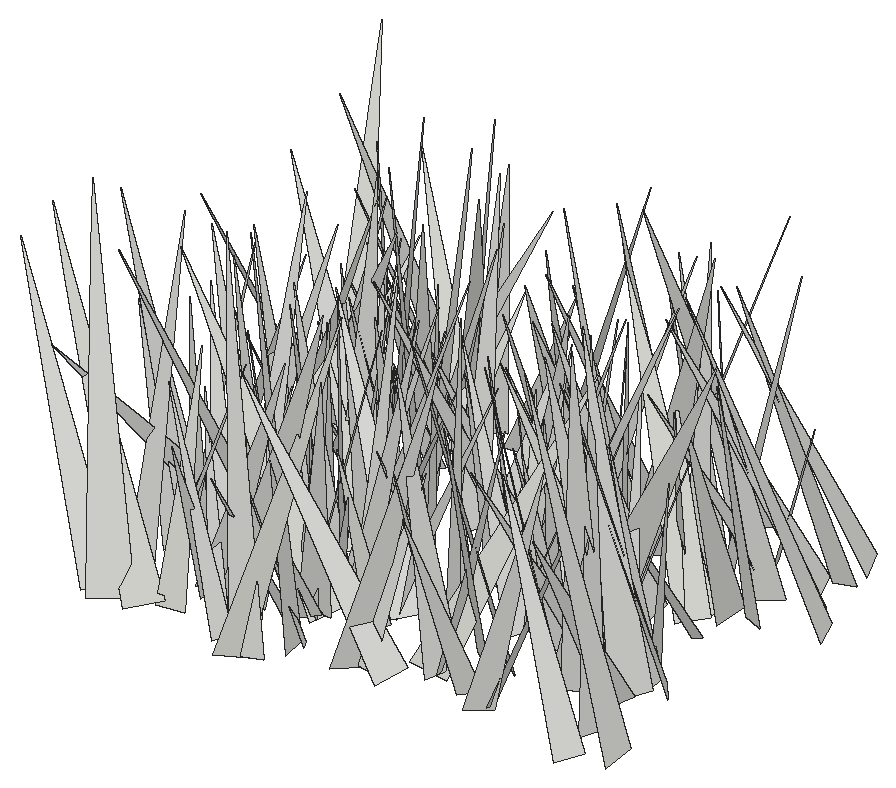
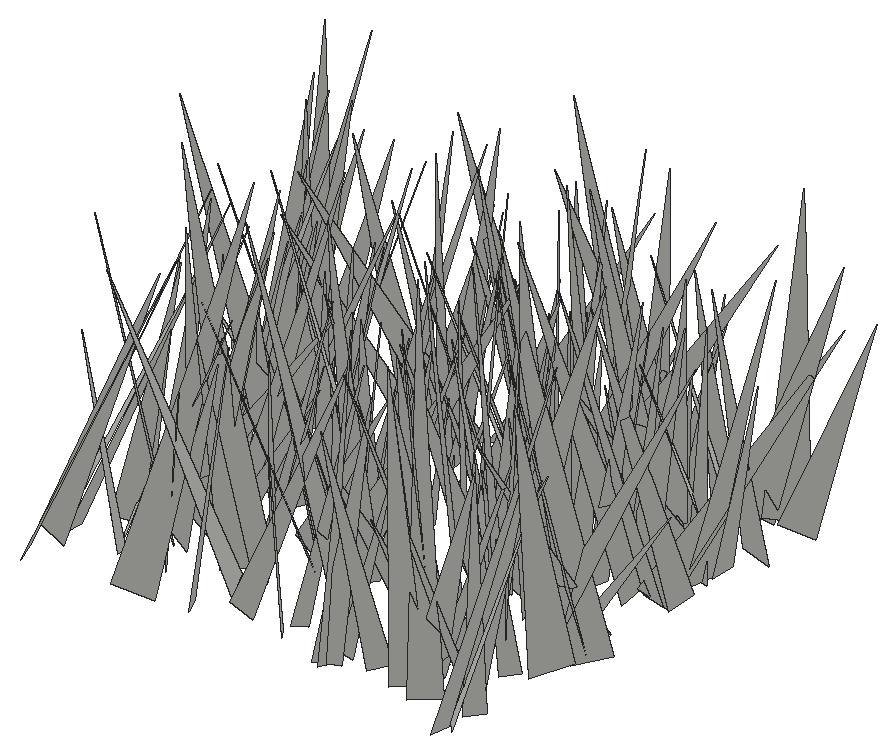
# SketchUp Ruby script. Lengths in inches.
U = 1.inch
M = Sketchup.active_model
def pt(a) = Geom::Point3d.new(a.map { |v| v * U })
def face(e, loops, mat)
  f = e.add_face(loops[0].map { |a| pt(a) })
  loops[1..].each { |l| e.add_face(l.map { |a| pt(a) }).erase! }
  f.material = f.back_material = mat if mat
  f
end
# faces: each face lists its corners as indices into pts; further lists are holes
def faces(e, pts, list, mat = nil) = list.each { |f| face(e, (f[0].is_a?(Array) ? f : [f]).map { |l| l.map { |i| pts[i] } }, mat) }
# xy, xz, yz: faces in a plane at the given z, y or x. An outline is a flat list of corners, or four numbers for a rectangle; further outlines are holes
def ring(l) = l.size == 4 ? [[l[0], l[1]], [l[2], l[1]], [l[2], l[3]], [l[0], l[3]]] : l.each_slice(2).to_a
def flat(e, list, mat, &to3) = list.each { |f| face(e, (f[0].is_a?(Array) ? f : [f]).map { |l| ring(l).map { |u, v| to3.(u, v) } }, mat) }
def xy(e, z, list, mat = nil) = flat(e, list, mat) { |x, y| [x, y, z] }
def xz(e, y, list, mat = nil) = flat(e, list, mat) { |x, z| [x, y, z] }
def yz(e, x, list, mat = nil) = flat(e, list, mat) { |y, z| [x, y, z] }
def lines(e, pts, list) = list.each { |a, b| e.add_line(pt(pts[a]), pt(pts[b])) }
# prism: a flat outline (further loops are holes) pulled along v
def prism(e, loops, v, mat = nil)
  f = face(e, loops, mat); d = Geom::Vector3d.new(v.map { |x| x * U })
  f.pushpull(f.normal.samedirection?(d) ? d.length : -d.length)
end
def box(e, o, s, mat = nil) = prism(e, [[o, [o[0] + s[0], o[1], o[2]], [o[0] + s[0], o[1] + s[1], o[2]], [o[0], o[1] + s[1], o[2]]]], [0, 0, s[2]], mat)
def at(x, y, z, deg = 0) = Geom::Transformation.translation(pt([x, y, z])) * Geom::Transformation.rotation(ORIGIN, Z_AXIS, deg.degrees)
def axes(o, x, y, z) = Geom::Transformation.new([*x, 0, *y, 0, *z, 0, *pt(o).to_a, 1])
def part(name) = M.definitions.add(name)
# library, detail: a bought-in or finely detailed component or shape, given as its bounding box
def library(name, o, s) = part(name).tap { |d| box(d.entities, o, s) }
def detail(e, o, s) = box(e.add_group.entities, o, s)
def put(e, d, t, mat = nil) = e.add_instance(d, t).tap { |i| i.material = mat if mat }
def group(e, t, mat = nil) = e.add_group.tap { |g| g.transformation = t; g.material = mat if mat }.entities
root = M.entities
c1 = part("fur_instance\#9")
p = [[0.8125,0,1.79],[0.67,-0.02,1.48],[0,-0.11,0],[0,0.11,0]]
faces(c1.entities,p,[[0,1,2,3]])
put(root,c1,axes([68.28,290.38,-27.1],[4.10212,-1.60455,0.85508],[-1.23063,-4.00368,-1.60913],[-1.3384,-1.23658,4.10033]))
put(root,c1,axes([70.8,287.91,-27.1],[-4.9286,0.63717,0.02707],[0.62924,4.89286,-0.60144],[0.10377,0.59304,4.93308]))
put(root,c1,axes([65.69,287.62,-27.1],[-4.19179,6.94453,1.88873],[7.18228,4.17546,0.58769],[0.45687,-1.92457,8.09026]))
put(root,c1,axes([80.6,290.35,-27.1],[1.77342,-4.13167,0.71101],[-4.001,-1.89854,-1.053],[-1.2523,0.21471,4.37115]))
put(root,c1,axes([77.55,289.49,-27.1],[-6.03456,2.61232,0.13904],[2.52964,5.73798,1.98392],[-0.66667,-1.87372,6.2693]))
put(root,c1,axes([71.93,286.99,-27.1],[6.32729,-2.1008,2.73388],[-3.01636,-6.1404,2.26257],[-1.67006,3.13117,6.27127]))
put(root,c1,axes([86.57,288.8,-27.1],[-4.85696,2.92878,0.85344],[3.03677,4.79447,0.82904],[0.29007,-1.15391,5.61075]))
put(root,c1,axes([72.45,287.27,-27.1],[0.0482,8.00911,1.76337],[7.92916,-0.49572,2.03478],[-2.09374,-1.69294,7.74648]))
put(root,c1,axes([72.46,290.14,-27.1],[-0.70477,-3.63934,0.22038],[-3.52996,0.62491,-0.96896],[-0.91253,0.39339,3.57807]))
put(root,c1,axes([67.9375,288.38,-27.1],[-1.16882,5.10436,1.64073],[5.31118,1.33199,-0.3603],[0.7334,-1.51127,5.22406]))
put(root,c1,axes([64.84,288.08,-27.1],[-3.24359,5.98487,0.42852],[5.75195,2.96279,2.1587],[-1.708,-1.38792,6.45597]))
put(root,c1,axes([66.96,288.01,-27.1],[-3.17251,7.14398,0.8627],[6.87917,2.73438,2.65436],[-2.11131,-1.82544,7.35225]))
put(root,c1,axes([73.53,289.39,-27.1],[-3.08913,-1.9262,0.20442],[-1.91689,2.98464,-0.84391],[-0.27849,0.82245,3.5413]))
put(root,c1,axes([69.64,290.49,-27.1],[3.88235,-7.18309,1.19208],[-7.15051,-3.50623,2.16032],[1.37403,2.04942,7.87416]))
put(root,c1,axes([75.89,289.04,-27.1],[6.31096,-2.97385,1.65761],[-3.28181,-6.24286,1.29466],[-0.9062,1.89806,6.85536]))
put(root,c1,axes([66.57,289.49,-27.1],[4.70564,3.18962,0.73071],[3.27223,-4.59158,-1.02983],[-0.01227,-1.26267,5.59072]))
put(root,c1,axes([87.99,289.93,-27.1],[-7.83982,-0.95667,1.33619],[-0.96404,7.9519,0.03699],[1.33088,0.12461,7.89789]))
put(root,c1,axes([81.66,289.57,-27.1],[4.65487,-3.05281,1.35089],[-3.29302,-4.57961,0.99778],[-0.54826,1.58741,5.47649]))
put(root,c1,axes([73.37,288.93,-27.1],[-7.60319,-2.30719,2.08818],[-2.71089,7.61771,-1.45385],[1.52798,2.03457,7.8114]))
put(root,c1,axes([76.24,289.36,-27.1],[-0.49271,4.25835,1.65602],[4.30491,0.99075,-1.26683],[1.53091,-1.41548,4.0953]))
put(root,c1,axes([68.3,290.51,-27.1],[3.9818,-4.86666,0.84742],[-4.90357,-3.76221,1.43455],[0.59785,1.55519,6.12218]))
put(root,c1,axes([78.86,290.92,-27.1],[-5.74569,2.33772,2.68731],[2.89131,6.03979,0.92776],[2.08013,-1.9379,6.13328]))
put(root,c1,axes([72.27,291.53,-27.1],[1.6892,-5.96403,1.00433],[-6.01842,-1.55459,0.89085],[0.59746,1.20222,6.13428]))
put(root,c1,axes([85.42,293.22,-27.1],[4.02503,-3.95124,0.17731],[-3.62061,-3.78264,-2.10414],[-1.59215,-1.38705,5.23314]))
put(root,c1,axes([77.93,292.04,-27.1],[-3.99319,-2.60087,1.40659],[-2.16034,4.18012,1.59628],[2.0189,-0.6713,4.49021]))
put(root,c1,axes([69.52,289.24,-27.1],[-0.27528,4.26527,0.41219],[4.05575,0.12601,1.40472],[-1.38323,-0.47937,4.03672]))
put(root,c1,axes([72.34,291.2,-27.1],[-3.051,-7.21191,1.32168],[-6.61753,2.09219,-3.8598],[-3.15701,2.58422,6.81338]))
put(root,c1,axes([79.625,292.39,-27.1],[-2.94569,-5.43055,1.36405],[-5.282,3.20651,1.35919],[1.85796,0.50597,6.02666]))
put(root,c1,axes([74.94,292.03,-27.1],[3.15907,-2.58161,1.45094],[-2.40771,-3.47422,-0.93937],[-1.72421,0.12146,3.97014]))
put(root,c1,axes([71.92,291.46,-27.1],[2.13967,5.72529,2.72362],[6.33838,-1.99885,-0.77766],[-0.14822,-2.82858,6.06237]))
put(root,c1,axes([72.78,291.84,-27.1],[-6.95314,3.37085,0.59923],[3.40426,6.66259,2.02209],[-0.36434,-2.07731,7.45788]))
put(root,c1,axes([72.22,292.96,-27.1],[-0.71595,-3.844,0.50308],[-3.36107,0.87042,1.86752],[1.93201,0.08975,3.4353]))
put(root,c1,axes([68.78,290.76,-27.1],[3.00603,-4.02582,3.59921],[-4.80148,-3.87769,-0.32715],[-2.47129,2.63706,5.01362]))
put(root,c1,axes([78.77,291.2,-27.1],[5.20805,0.62891,1.21236],[0.54515,-5.33937,0.42794],[-1.25226,0.29119,5.2284]))
put(root,c1,axes([65.85,295.35,-27.1],[3.04305,-5.48081,0.27728],[-4.42438,-2.6378,-3.58374],[-3.24669,-1.54241,5.14356]))
put(root,c1,axes([80.59,292.77,-27.1],[-4.6315,-5.30606,1.24554],[-5.44783,4.55599,-0.84886],[0.16366,1.49838,6.99175]))
put(root,c1,axes([83.85,293.1,-27.1],[3.80262,-6.94068,2.14426],[-7.19034,-3.9408,-0.00453],[-1.0344,1.87826,7.9141]))
put(root,c1,axes([70.47,289.55,-27.1],[0.64716,8.27924,1.09317],[8.31403,-0.74193,0.69715],[-0.78591,-1.0312,8.27518]))
put(root,c1,axes([71.38,292.79,-27.1],[2.3019,2.88607,2.09295],[3.52279,-2.224,-0.8077],[-0.54756,-2.17555,3.60219]))
put(root,c1,axes([64.86,290.47,-27.1],[1.29784,6.7007,1.25957],[6.74597,-1.44798,0.75208],[-0.98888,-1.08363,6.78367]))
put(root,c1,axes([81.89,295.59,-27.1],[-4.9139,-3.74374,0.55427],[-3.15126,4.55055,2.79845],[2.0958,-1.9355,5.50733]))
put(root,c1,axes([78.78,291.56,-27.1],[2.86323,5.98862,2.41998],[6.20716,-3.28322,0.78076],[-1.78634,-1.80966,6.59182]))
put(root,c1,axes([86.06,290.8125,-27.1],[-7.47088,0.3057,1.86762],[-0.12287,7.51123,-1.721],[1.88848,1.69808,7.27638]))
put(root,c1,axes([82.6,293.33,-27.1],[0.98375,-3.96673,0.69714],[-3.91068,-0.76919,1.14174],[0.96305,0.9285,3.92417]))
put(root,c1,axes([77.86,292.07,-27.1],[-5.58164,-0.15602,0.84627],[-0.25003,5.60842,-0.61509],[0.82341,0.64537,5.54984]))
put(root,c1,axes([70.68,294.19,-27.1],[-2.8459,-6.01928,1.64103],[-5.98512,3.14324,1.14988],[1.76154,0.95508,6.5581]))
put(root,c1,axes([73.4,292.625,-27.1],[2.35807,6.09522,2.44102],[6.53945,-1.94795,-1.45322],[0.58808,-2.77931,6.37184]))
put(root,c1,axes([81.83,290.06,-27.1],[5.28462,2.45266,0.54887],[2.09175,-5.00051,2.20534],[-1.39334,1.79538,5.39252]))
put(root,c1,axes([65.07,292.19,-27.1],[-4.79431,0.50788,0.77321],[0.45097,4.84644,-0.38709],[0.80772,0.30866,4.80557]))
put(root,c1,axes([82.95,292.87,-27.1],[-4.95008,-4.07189,1.35786],[-4.2827,4.82407,-1.14641],[0.2873,1.75371,6.30629]))
put(root,c1,axes([65.53,293.16,-27.1],[1.09401,4.63876,2.44173],[5.21296,-1.22556,-0.00737],[-0.55243,-2.37843,4.76601]))
put(root,c1,axes([78.37,290.66,-27.1],[-2.47927,6.31853,1.78834],[5.49074,3.04318,-3.14001],[3.60191,-0.28983,6.01756]))
put(root,c1,axes([65.26,293.36,-27.1],[-7.08698,0.49693,1.41438],[0.58095,7.2106,0.37757],[1.38199,-0.48283,7.09434]))
put(root,c1,axes([84.66,293.85,-27.1],[-2.85824,2.70123,1.97363],[3.21945,2.92659,0.65696],[0.90938,-1.87078,3.87745]))
put(root,c1,axes([68.97,293.72,-27.1],[3.31439,2.62679,2.62231],[3.03004,-3.94532,0.12232],[-2.14367,-1.5153,4.22732]))
put(root,c1,axes([75.84,294.84,-27.1],[-3.61169,-1.5954,0.61372],[-1.41522,3.59542,1.01805],[0.9587,-0.70282,3.81487]))
put(root,c1,axes([85.44,293.875,-27.1],[-6.5147,3.53544,2.59254],[3.94464,6.75335,0.70282],[1.91322,-1.88542,7.3788]))
put(root,c1,axes([71.05,294.2,-27.1],[1.22573,-5.85041,2.29876],[-6.17569,-1.55733,-0.67049],[-1.1715,2.08841,5.93971]))
put(root,c1,axes([83.51,294.98,-27.1],[3.66547,-5.8791,2.24711],[-5.89364,-4.11869,-1.16204],[-2.20868,1.23351,6.83002]))
put(root,c1,axes([71,294.77,-27.1],[5.57047,2.74276,2.66238],[3.42235,-5.67452,-1.31471],[-1.7025,-2.43273,6.06831]))
put(root,c1,axes([74.32,293.71,-27.1],[4.41432,4.17138,0.78555],[4.1779,-4.06951,-1.86761],[0.75011,-1.88212,5.77916]))
put(root,c1,axes([67.03,291.81,-27.1],[-1.28039,5.01222,0.36244],[4.5705,1.31696,-2.06622],[2.08908,0.19072,4.74262]))
put(root,c1,axes([84.68,296.38,-27.1],[-3.9391,-6.11846,0.96009],[-6.01065,4.05101,1.1555],[1.49311,0.1661,7.18449]))
put(root,c1,axes([81.25,295,-27.1],[0.8668,-4.44855,1.11397],[-4.54098,-0.99091,-0.42373],[-0.6404,1.00517,4.51236]))
put(root,c1,axes([86.24,295.04,-27.1],[-5.08924,-4.37631,0.84531],[-4.44671,5.07308,-0.50754],[0.30556,0.93743,6.69289]))
put(root,c1,axes([66.2,291.19,-27.1],[3.80784,5.11048,0.67094],[4.57882,-3.73693,2.47721],[-2.36675,0.99257,5.87197]))
put(root,c1,axes([67.23,294.42,-27.1],[1.7878,3.1828,1.34143],[3.44443,-1.53093,-0.95817],[0.2561,-1.62848,3.52255]))
put(root,c1,axes([73.9,292.28,-27.1],[1.51119,6.34193,0.92742],[6.21067,-1.68435,1.39797],[-1.58356,-0.55387,6.36784]))
put(root,c1,axes([70.28,294.2,-27.1],[5.04239,2.3615,1.06864],[2.46365,-5.09289,-0.37039],[-0.80566,-0.79378,5.55564]))
put(root,c1,axes([75.21,293.49,-27.1],[-4.13597,4.87198,0.25098],[4.78591,3.98836,1.44689],[-0.94567,-1.12348,6.22487]))
put(root,c1,axes([67.33,294.07,-27.1],[-1.25475,3.57203,1.31412],[3.70812,1.4592,-0.42579],[0.858,-1.08261,3.76198]))
put(root,c1,axes([80.79,296.01,-27.1],[-3.85431,-2.63258,1.04926],[-2.43046,3.98156,1.06172],[1.4575,-0.32233,4.54521]))
put(root,c1,axes([67.47,294.52,-27.1],[4.90342,0.51596,3.18153],[0.4361,-5.84514,0.27581],[-3.19346,-0.00597,4.92277]))
put(root,c1,axes([67.18,294.54,-27.1],[-2.59565,5.50063,1.7013],[5.74289,2.3395,1.19781],[-0.41302,-2.03926,5.96319]))
put(root,c1,axes([69.4,295.45,-27.1],[-3.39336,2.50243,2.08506],[2.97495,3.60715,0.51243],[1.32637,-1.68843,4.18502]))
put(root,c1,axes([70.04,295.3,-27.1],[-2.18081,-4.36379,1.96245],[-4.63729,2.45895,0.31456],[1.17875,1.60022,4.86823]))
put(root,c1,axes([85.58,295.17,-27.1],[-4.70558,-0.80345,0.83315],[-0.88013,4.74917,-0.39105],[0.7517,0.53106,4.75763]))
put(root,c1,axes([64.83,294.93,-27.1],[6.22243,-0.20354,0.93497],[-0.30289,-6.25415,0.65425],[-0.90767,0.69164,6.19128]))
put(root,c1,axes([79.24,295,-27.1],[-5.48361,2.04542,0.49712],[2.0602,5.49974,0.09665],[0.43181,-0.2646,5.85187]))
put(root,c1,axes([82.76,296.75,-27.1],[-6.27523,-0.24227,0.55286],[-0.1392,6.19931,1.13667],[0.58735,-1.11924,6.17618]))
put(root,c1,axes([79.81,296.55,-27.1],[-0.67343,-4.75938,1.30258],[-4.88536,0.82798,0.49956],[0.69398,1.21023,4.78075]))
put(root,c1,axes([84.96,295.9,-27.1],[4.07501,0.67414,1.38281],[0.80205,-4.27202,-0.28088],[-1.31276,-0.5174,4.12083]))
put(root,c1,axes([68.17,295.95,-27.1],[-6.22894,0.57755,1.75246],[0.68588,6.45268,0.31131],[1.71297,-0.48351,6.24791]))
put(root,c1,axes([71.85,294.54,-27.1],[4.96936,4.425,0.65774],[4.44372,-4.99597,0.03757],[-0.51632,-0.4092,6.65385]))
put(root,c1,axes([72.39,294.59,-27.1],[-5.98582,-0.44068,0.88109],[-0.67667,5.78235,-1.70504],[0.71598,1.78068,5.75475]))
put(root,c1,axes([71.47,294.6875,-27.1],[3.13584,4.70476,0.63652],[4.72939,-3.16238,0.0748],[-0.41563,-0.48786,5.65355]))
put(root,c1,axes([65.77,295.44,-27.1],[2.77668,6.00015,1.42785],[6.14966,-2.57364,-1.14395],[0.47149,-1.76779,6.51177]))
put(root,c1,axes([83.8125,294.18,-27.1],[3.6245,2.89722,0.22495],[2.66528,-3.45765,1.58821],[-1.15791,1.11007,4.35987]))
put(root,c1,axes([66.61,295.44,-27.1],[7.58645,0.4489,1.20084],[0.2907,-7.62155,1.01257],[-1.24861,0.95304,7.53196]))
put(root,c1,axes([71.38,296.2,-27.1],[-4.19942,1.95994,0.17006],[1.96728,4.18576,0.33862],[0.01038,-0.37878,4.62189]))
put(root,c1,axes([70.23,297.34,-27.1],[-1.89592,-3.45095,1.30694],[-3.60556,2.04518,0.16982],[0.78554,1.05823,3.9338]))
put(root,c1,axes([78.68,296.26,-27.1],[-1.71851,4.03919,1.0736],[4.16688,1.74577,0.10182],[0.32374,-1.02868,4.3884]))
put(root,c1,axes([80.59,298.2,-27.1],[3.82613,-7.13137,0.63835],[-6.75778,-3.35774,2.99351],[2.36564,1.94225,7.51895]))
put(root,c1,axes([70.69,298.54,-27.1],[1.15457,-5.41906,0.82486],[-5.48032,-1.12384,0.28761],[0.11275,0.86626,5.53322]))
put(root,c1,axes([70.06,296.42,-27.1],[-4.21577,-3.58718,3.5566],[-4.31781,4.96325,-0.11214],[2.62178,2.40587,5.53425]))
put(root,c1,axes([77.64,297.25,-27.1],[-3.40834,-0.81843,0.94444],[-0.85751,3.5273,-0.03792],[0.90911,0.25869,3.50503]))
put(root,c1,axes([75.55,296.52,-27.1],[-3.65849,-0.26653,0.63033],[-0.40108,3.61269,-0.80033],[0.55452,0.85461,3.57982]))
put(root,c1,axes([78.79,295.35,-27.1],[1.97963,5.14738,0.61551],[5.06452,-2.06097,0.94673],[-1.10678,-0.22402,5.43306]))
put(root,c1,axes([77.17,298.64,-27.1],[-0.65869,-6.64833,1.3688],[-6.16249,0.00919,-2.92087],[-2.84565,1.51902,6.00855]))
put(root,c1,axes([77.3,298.23,-27.1],[4.68379,1.41709,0.13919],[1.37897,-4.39495,-1.65779],[0.35492,-1.62533,4.60411]))
put(root,c1,axes([76.19,297.3,-27.1],[-1.43157,-3.77915,1.63266],[-4.11341,1.2436,-0.72817],[-0.16553,1.78,3.97506]))
put(root,c1,axes([84.27,295.07,-27.1],[0.39127,5.5531,0.09038],[5.24022,-0.39914,1.8382],[-1.83989,0.04412,5.25462]))
put(root,c1,axes([69.49,297.36,-27.1],[6.01123,-4.10409,2.83515],[-4.50522,-6.3728,0.32708],[-2.14119,1.8869,7.27128]))
put(root,c1,axes([82.32,299.1,-27.1],[-6.75805,0.02177,1.99006],[0.56326,6.77748,1.83863],[1.90881,-1.92284,6.50317]))
put(root,c1,axes([71.15,297.3125,-27.1],[4.07736,0.20577,0.16386],[0.20057,-4.0788,0.13116],[-0.17019,0.12285,4.08044]))
put(root,c1,axes([77.86,297.69,-27.1],[-3.21218,-2.63282,1.4726],[-2.81239,3.39173,-0.07071],[1.09119,0.99138,4.15269]))
put(root,c1,axes([77.29,297.56,-27.1],[6.01088,3.96881,0.98389],[4.08835,-5.80352,-1.56674],[0.06989,-1.84874,7.03046]))
put(root,c1,axes([77.79,296.9,-27.1],[1.94279,3.86541,2.10519],[3.74501,-2.66073,1.42935],[-2.3126,-1.06149,4.08323]))
put(root,c1,axes([70.67,296.16,-27.1],[-2.92778,3.00983,0.00711],[2.98882,2.90849,-0.48849],[0.35507,0.33555,4.17041]))
put(root,c1,axes([70.76,297.41,-27.1],[-6.11884,4.72961,1.11538],[4.85918,5.97068,1.339],[0.0418,-1.7422,7.61686]))
put(root,c1,axes([72,298.42,-27.1],[-6.4664,-4.252,2.80304],[-4.40658,6.94256,0.3657],[2.55316,1.21333,7.73047]))
put(root,c1,axes([70.33,299.01,-27.1],[-1.26664,-5.03308,1.07763],[-5.14261,1.28411,-0.04714],[0.2163,1.05675,5.1898]))
put(root,c1,axes([84.58,298.9,-27.1],[-2.08934,-4.39389,0.06996],[-3.98317,1.86084,-2.08523],[-1.85622,0.95264,4.39584]))
put(root,c1,axes([78.07,299.7,-27.1],[4.2644,-2.86076,0.08373],[-2.8192,-4.22473,-0.76148],[-0.49304,-0.58632,5.07831]))
put(root,c1,axes([72.58,298.06,-27.1],[-3.23296,-4.09809,2.47034],[-4.47809,3.64184,0.18098],[1.68632,1.81429,5.21667]))
put(root,c1,axes([64.67,300.42,-27.1],[3.10816,-7.62871,0.22312],[-7.12075,-2.81203,3.04879],[2.74626,1.34273,7.65263]))
put(root,c1,axes([69.96,299.4,-27.1],[5.00049,1.26706,0.71261],[1.41038,-4.84715,-1.27832],[-0.35226,-1.4205,4.99762]))
put(root,c1,axes([84.55,300.92,-27.1],[5.34642,-2.10558,1.0321],[-1.67954,-5.23165,-1.97278],[-1.63641,-1.50973,5.39684]))
put(root,c1,axes([74.78,300.79,-27.1],[-4.80536,-1.45342,1.08645],[-0.98448,4.67157,1.89512],[1.52434,-1.5647,4.64891]))
put(root,c1,axes([67.03,300.47,-27.1],[-2.83632,-6.0499,0.28173],[-5.90232,2.69141,-1.62612],[-1.35766,0.93829,6.48088]))
put(root,c1,axes([77.51,299.02,-27.1],[5.84897,4.9177,0.90335],[4.92852,-5.43629,-2.31659],[0.84231,-2.33947,7.282]))
put(root,c1,axes([75.44,300.46,-27.1],[0.87943,-6.58228,1.27772],[-6.45662,-0.48373,1.95201],[1.80858,1.47376,6.34739]))
put(root,c1,axes([66.375,299.27,-27.1],[-2.80536,-2.90649,0.0794],[-2.63209,2.49174,-1.78533],[-1.23535,1.29136,3.62358]))
put(root,c1,axes([78.66,297.89,-27.1],[-2.98771,2.56269,0.00271],[2.54357,2.96592,-0.47684],[0.31249,0.36018,3.90722]))
put(root,c1,axes([69.94,298.18,-27.1],[0.78619,5.10987,0.99795],[4.99569,-1.02461,1.31074],[-1.46621,-0.75112,5.00108]))
put(root,c1,axes([81.87,299.65,-27.1],[-2.56697,2.61634,0.35758],[2.51502,2.27032,1.44317],[-0.80484,-1.25014,3.36925]))
put(root,c1,axes([82.16,301.13,-27.1],[-2.28168,-4.43341,1.38047],[-4.1851,2.6298,1.52839],[2.0114,0.44265,4.74608]))
put(root,c1,axes([78.6,300.17,-27.1],[-1.09532,-3.977,1.33167],[-3.82769,0.38536,-1.99748],[-1.71426,1.68065,3.6092]))
put(root,c1,axes([68.92,298.85,-27.1],[-4.7564,-0.43454,1.78324],[-0.95829,4.81251,-1.3833],[1.56539,1.62573,4.5715]))
put(root,c1,axes([71.18,298.6,-27.1],[5.70541,0.17051,1.69377],[-0.31532,-5.71566,1.63753],[-1.67287,1.65887,5.46803]))
put(root,c1,axes([85.47,301.08,-27.1],[-2.10468,-4.52268,1.53831],[-4.75533,2.14388,-0.20306],[0.45584,1.48319,4.98428]))
put(root,c1,axes([84.18,303.81,-27.1],[-4.88167,-3.98465,0.29136],[-3.56929,4.55624,2.50876],[1.79514,-1.77658,5.7805]))
put(root,c1,axes([65.35,300.1,-27.1],[3.97347,4.57155,1.31094],[4.73936,-3.94824,-0.59665],[-0.39506,-1.38509,6.02757]))
put(root,c1,axes([83.66,299.96,-27.1],[-6.02819,4.2729,0.70004],[4.32885,5.97346,0.81585],[0.09372,-1.07093,7.34378]))
put(root,c1,axes([83.77,299.96,-27.1],[-3.58743,2.64736,0.43412],[2.66538,3.59954,0.07504],[0.30449,-0.3184,4.45786]))
put(root,c1,axes([65.8,298.71,-27.1],[-0.63862,5.35473,0.03552],[5.1577,0.62471,-1.44573],[1.43964,0.13724,5.19527]))
put(root,c1,axes([88.13,302.13,-27.1],[-6.75441,-2.93713,0.31923],[-2.94167,6.75982,-0.04619],[0.27431,0.1697,7.36523]))
put(root,c1,axes([82.39,301.57,-27.1],[1.71463,6.79892,3.94816],[7.36353,-2.80488,1.63226],[-2.7553,-3.26505,6.81916]))
put(root,c1,axes([79.28,302.54,-27.1],[6.86151,-4.43995,0.81428],[-4.49635,-6.85344,0.51929],[-0.39875,0.87961,8.15621]))
put(root,c1,axes([80.11,300.33,-27.1],[-7.13799,-1.18277,0.6594],[-1.323,6.84565,-2.04241],[0.28881,2.12669,6.94107]))
put(root,c1,axes([84.92,302.84,-27.1],[1.57492,-4.967,1.49516],[-5.0252,-1.8484,-0.84719],[-1.28605,1.13987,5.14138]))
put(root,c1,axes([67.52,302.09,-27.1],[6.90611,3.10223,2.59996],[3.46907,-7.18559,-0.64093],[-2.08547,-1.6797,7.5437]))
put(root,c1,axes([77.62,300.59,-27.1],[2.96652,3.66752,1.13191],[3.55325,-3.16507,0.94281],[-1.45132,-0.25254,4.62191]))
put(root,c1,axes([86.01,304.54,-27.1],[-6.75502,-2.37628,0.59319],[-2.11002,6.52988,2.13012],[1.24354,-1.82836,6.83664]))
put(root,c1,axes([69.31,302.26,-27.1],[-4.14785,-5.45032,3.6874],[-5.74845,5.12259,1.10541],[3.20285,2.13555,6.75935]))
put(root,c1,axes([68.98,302.9375,-27.1],[-0.44719,-4.16584,0.88919],[-4.01944,0.11666,-1.47491],[-1.41032,0.98845,3.92158]))
put(root,c1,axes([82.84,300.96,-27.1],[0.75585,6.87514,1.87347],[7.05211,-0.99202,0.79528],[-1.02238,-1.75986,6.87069]))
put(root,c1,axes([72.99,300.08,-27.1],[-6.34351,2.24327,1.15963],[1.89857,6.30395,-1.80908],[1.66506,1.35834,6.48071]))
put(root,c1,axes([78.98,301.5,-27.1],[3.80015,2.05854,2.10545],[1.83657,-4.34391,0.93228],[-2.30164,-0.0674,4.22014]))
put(root,c1,axes([67.35,302.51,-27.1],[-4.34525,-4.69158,2.51984],[-5.05188,4.66036,-0.03462],[1.68493,1.87398,6.3946]))
put(root,c1,axes([66.38,303.16,-27.1],[3.1539,-2.32332,0.00557],[-2.32207,-3.15188,0.13648],[0.07647,0.11319,3.91488]))
put(root,c1,axes([87.12,303.24,-27.1],[-4.6266,-2.97065,0.07987],[-2.96143,4.59663,-0.58091],[-0.24706,0.53178,5.46742]))
put(root,c1,axes([73.64,300.59,-27.1],[-2.96386,2.60362,0.59977],[2.15648,2.85999,-1.75873],[1.5774,0.98217,3.53132]))
put(root,c1,axes([71.88,300.91,-27.1],[4.93577,0.48548,2.66433],[-0.37318,-5.36398,1.66873],[-2.68236,1.63958,4.67042]))
put(root,c1,axes([77.28,301.3125,-27.1],[4.12664,4.96749,0.53315],[4.97839,-4.14664,0.10195],[-0.41933,-0.34468,6.45715]))
put(root,c1,axes([74.79,305.16,-27.1],[4.72297,-1.05883,1.70864],[-0.28791,-4.67444,-2.10088],[-1.98939,-1.83725,4.36049]))
put(root,c1,axes([68.6,304.61,-27.1],[-1.93771,-4.14246,0.35212],[-4.15628,1.93921,-0.05843],[0.0961,0.34375,4.57288]))
put(root,c1,axes([73.93,303.43,-27.1],[7.81228,1.65656,1.00866],[1.73052,-7.84393,-0.52089],[-0.87571,-0.72239,7.96898]))
put(root,c1,axes([82.75,302.88,-27.1],[4.81614,4.80746,1.57054],[5.00941,-4.83285,-0.56818],[-0.69571,-1.51836,6.78115]))
put(root,c1,axes([77.59,303.97,-27.1],[-4.87581,-1.54153,0.97742],[-1.54685,4.96967,0.12147],[0.96896,0.17664,5.11224]))
put(root,c1,axes([67.71,306.55,-27.1],[7.63705,-2.12328,0.08153],[-2.0044,-7.29978,-2.35267],[-0.70524,-2.24596,7.56953]))
put(root,c1,axes([84.01,303.14,-27.1],[-6.46685,-0.99912,0.02995],[-0.985,6.33639,-1.3035],[-0.17003,1.29271,6.41243]))
put(root,c1,axes([79.42,303.23,-27.1],[-2.32023,4.26891,1.78267],[4.38145,2.66784,-0.68595],[1.48474,-1.20167,4.81004]))
put(root,c1,axes([77.23,305.58,-27.1],[-0.62326,-5.57048,0.69706],[-5.46922,0.44429,-1.33972],[-1.26641,0.82277,5.44278]))
put(root,c1,axes([83.5,304.85,-27.1],[4.06757,1.21437,0.51699],[1.31683,-3.847,-1.32426],[-0.08902,-1.4188,4.03313]))
put(root,c1,axes([81.27,307,-27.1],[1.71301,-8.16044,0.92704],[-8.06805,-1.84913,-1.36891],[-1.53583,0.61199,8.22516]))
put(root,c1,axes([66.06,306.11,-27.1],[1.11267,-4.69864,0.20362],[-4.67497,-1.12782,-0.47895],[-0.51316,0.0867,4.80478]))
put(root,c1,axes([69.54,303.9,-27.1],[4.78863,4.89843,2.46119],[5.13986,-5.14824,0.24599],[-1.90629,-1.57608,6.84581]))
put(root,c1,axes([72.25,306.86,-27.1],[5.97611,0.87511,2.00016],[1.66713,-5.59279,-2.53411],[-1.40966,-2.90435,5.48252]))
put(root,c1,axes([82.54,302.83,-27.1],[0.67019,6.07953,1.22269],[5.42193,-1.17133,2.85227],[-3.0097,-0.75637,5.41058]))
put(root,c1,axes([72.13,305.79,-27.1],[-0.71572,-3.67555,0.46048],[-3.70429,0.70984,-0.09154],[-0.00255,0.46948,3.74347]))
put(root,c1,axes([86.35,305.45,-27.1],[-1.63613,-6.00923,1.56488],[-6.02721,1.14742,-1.89548],[-1.49415,1.95172,5.93253]))
put(root,c1,axes([72.26,306.72,-27.1],[3.35364,-3.87615,0.32814],[-3.76663,-3.34394,-1.00479],[-0.97195,-0.41544,5.02611]))
put(root,c1,axes([65.37,301.95,-27.1],[-6.50457,4.89284,0.5628],[4.72218,6.46057,-1.59001],[1.39918,0.94188,7.98255]))
put(root,c1,axes([65.54,306.34,-27.1],[4.72712,-1.54603,0.79765],[-1.39638,-4.74943,-0.93014],[-1.03759,-0.65178,4.88576]))
put(root,c1,axes([66.53,305.34,-27.1],[3.98085,5.13777,1.04709],[4.9615,-3.26572,-2.83883],[1.69606,-2.50573,5.84679]))
put(root,c1,axes([70.51,305.75,-27.1],[2.89103,-3.61881,0.35286],[-3.55779,-2.72252,1.22815],[0.74997,1.03461,4.46604]))
put(root,c1,axes([86.23,307.1875,-27.1],[-6.15592,-2.89241,0.11132],[-2.84807,6.09927,0.98037],[0.51666,-0.84058,6.73054]))
put(root,c1,axes([68.85,304.21,-27.1],[-0.53064,3.51066,0.60828],[3.36851,0.69471,-1.0709],[1.16098,-0.41106,3.38519]))
put(root,c1,axes([78.89,306.45,-27.1],[-4.44854,-2.43941,1.67916],[-2.34276,4.75236,0.69742],[1.81157,0.15557,5.02532]))
put(root,c1,axes([68.83,306.18,-27.1],[3.92094,-4.8226,1.73149],[-5.06492,-3.97791,0.39007],[-0.77596,1.59628,6.20315]))
put(root,c1,axes([81.86,304.3,-27.1],[-4.19914,-2.372,1.71601],[-2.90919,3.71707,-1.98087],[0.32817,2.60017,4.39719]))
put(root,c1,axes([69.15,304.56,-27.1],[-3.00084,5.06154,0.45444],[5.0055,2.85272,1.2797],[-0.87785,-1.03611,5.74339]))
put(root,c1,axes([65.8125,308.06,-27.1],[-7.05336,-2.15617,1.71578],[-1.62887,7.06566,2.18314],[2.22256,-1.66441,7.04506]))
put(root,c1,axes([78.5625,304.2,-27.1],[6.55777,3.05775,0.67545],[3.00333,-6.58518,0.65252],[-0.88663,0.30968,7.20614]))
put(root,c1,axes([74.96,306.01,-27.1],[2.81827,1.89164,1.24112],[2.11841,-2.90244,-0.38665],[-0.79437,-1.02901,3.37216]))
put(root,c1,axes([65.68,307.54,-27.1],[-3.97352,-3.33663,0.47318],[-3.25036,3.98768,0.8243],[0.89005,-0.33346,5.12275]))
